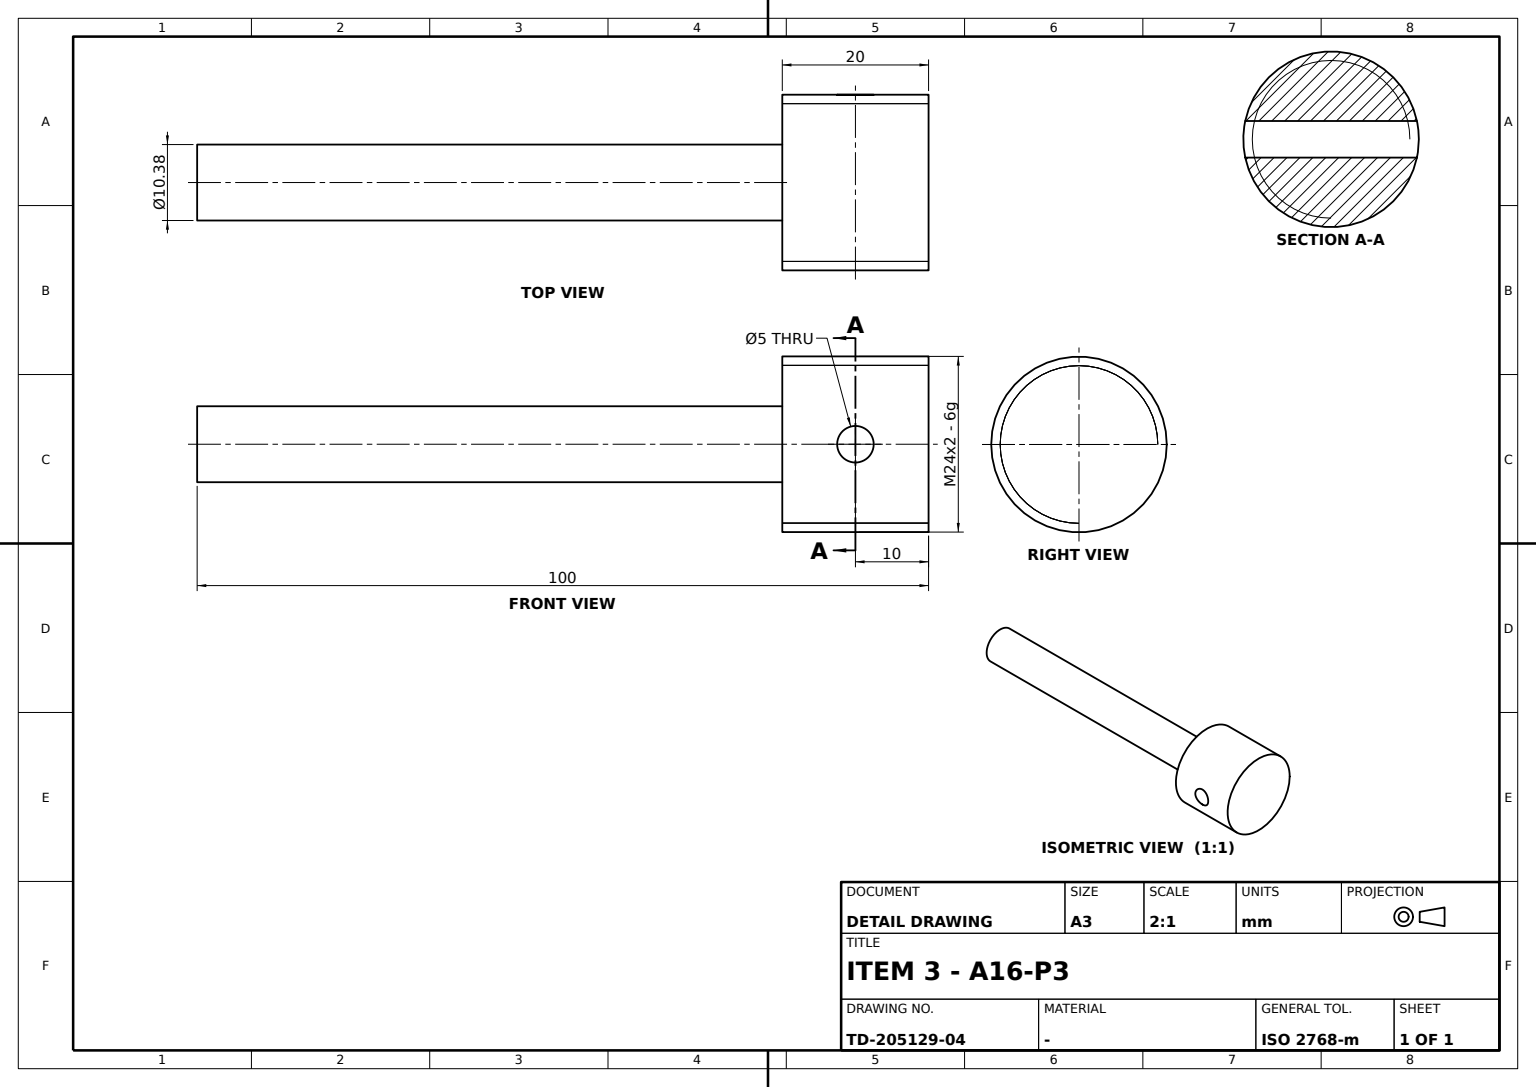
ISO-10303-21;
HEADER;
FILE_DESCRIPTION((''),'2;1');
FILE_NAME('','',(''),(''),'','','');
FILE_SCHEMA(('AUTOMOTIVE_DESIGN'));
ENDSEC;
DATA;
#1=APPLICATION_CONTEXT('');
#2=PRODUCT_CONTEXT('',#1,'mechanical');
#3=PRODUCT('','','',(#2));
#4=PRODUCT_DEFINITION_FORMATION('','',#3);
#5=PRODUCT_DEFINITION_CONTEXT('',#1,'design');
#6=PRODUCT_DEFINITION('','',#4,#5);
#7=PRODUCT_DEFINITION_SHAPE('','',#6);
#8=(LENGTH_UNIT()NAMED_UNIT(*)SI_UNIT(.MILLI.,.METRE.));
#9=(NAMED_UNIT(*)PLANE_ANGLE_UNIT()SI_UNIT($,.RADIAN.));
#10=(NAMED_UNIT(*)SI_UNIT($,.STERADIAN.)SOLID_ANGLE_UNIT());
#11=UNCERTAINTY_MEASURE_WITH_UNIT(LENGTH_MEASURE(0.005),#8,'distance_accuracy_value','');
#12=(GEOMETRIC_REPRESENTATION_CONTEXT(3)GLOBAL_UNCERTAINTY_ASSIGNED_CONTEXT((#11))GLOBAL_UNIT_ASSIGNED_CONTEXT((#8,#9,#10))REPRESENTATION_CONTEXT('',''));
#13=CARTESIAN_POINT('',(0.,12.,100.));
#14=VERTEX_POINT('',#13);
#15=CARTESIAN_POINT('',(0.,0.,100.));
#16=DIRECTION('',(0.,0.,-1.));
#17=DIRECTION('',(0.,1.,0.));
#18=AXIS2_PLACEMENT_3D('',#15,#16,#17);
#19=CIRCLE('',#18,12.);
#20=EDGE_CURVE('',#14,#14,#19,.T.);
#21=ORIENTED_EDGE('',*,*,#20,.F.);
#22=EDGE_LOOP('',(#21));
#23=FACE_BOUND('',#22,.T.);
#24=DIRECTION('',(1.,0.,0.));
#25=AXIS2_PLACEMENT_3D('',#13,#16,#24);
#26=PLANE('',#25);
#27=ADVANCED_FACE('',(#23),#26,.F.);
#28=CARTESIAN_POINT('',(0.,5.188,0.));
#29=VERTEX_POINT('',#28);
#30=CARTESIAN_POINT('',(0.,0.,0.));
#31=AXIS2_PLACEMENT_3D('',#30,#16,#17);
#32=CIRCLE('',#31,5.188);
#33=EDGE_CURVE('',#29,#29,#32,.T.);
#34=ORIENTED_EDGE('',*,*,#33,.F.);
#35=EDGE_LOOP('',(#34));
#36=FACE_BOUND('',#35,.T.);
#37=CARTESIAN_POINT('',(0.,5.188,80.));
#38=VERTEX_POINT('',#37);
#39=CARTESIAN_POINT('',(0.,0.,80.));
#40=AXIS2_PLACEMENT_3D('',#39,#16,#17);
#41=CIRCLE('',#40,5.188);
#42=EDGE_CURVE('',#38,#38,#41,.T.);
#43=ORIENTED_EDGE('',*,*,#42,.T.);
#44=EDGE_LOOP('',(#43));
#45=FACE_BOUND('',#44,.T.);
#46=CARTESIAN_POINT('',(0.,0.,50.));
#47=AXIS2_PLACEMENT_3D('',#46,#16,#24);
#48=CYLINDRICAL_SURFACE('',#47,5.188);
#49=ADVANCED_FACE('',(#36,#45),#48,.T.);
#50=ORIENTED_EDGE('',*,*,#33,.T.);
#51=EDGE_LOOP('',(#50));
#52=FACE_BOUND('',#51,.T.);
#53=AXIS2_PLACEMENT_3D('',#30,#16,#24);
#54=PLANE('',#53);
#55=ADVANCED_FACE('',(#52),#54,.T.);
#56=ORIENTED_EDGE('',*,*,#42,.F.);
#57=EDGE_LOOP('',(#56));
#58=FACE_BOUND('',#57,.T.);
#59=CARTESIAN_POINT('',(0.,12.,80.));
#60=VERTEX_POINT('',#59);
#61=CIRCLE('',#40,12.);
#62=EDGE_CURVE('',#60,#60,#61,.T.);
#63=ORIENTED_EDGE('',*,*,#62,.T.);
#64=EDGE_LOOP('',(#63));
#65=FACE_BOUND('',#64,.T.);
#66=AXIS2_PLACEMENT_3D('',#37,#16,#24);
#67=PLANE('',#66);
#68=ADVANCED_FACE('',(#58,#65),#67,.T.);
#69=CARTESIAN_POINT('',(2.5,-11.736695,90.));
#70=VERTEX_POINT('',#69);
#71=CARTESIAN_POINT('',(1.958372,-11.870043,91.960573));
#72=CARTESIAN_POINT('',(2.770873,-11.670071,89.999616));
#73=CARTESIAN_POINT('',(1.958134,-11.869843,88.040963));
#74=CARTESIAN_POINT('',(0.003168,-12.065028,87.229905));
#75=CARTESIAN_POINT('',(-1.958354,-11.870046,88.03942));
#76=CARTESIAN_POINT('',(-2.770873,-11.670071,90.000335));
#77=CARTESIAN_POINT('',(-1.958152,-11.869839,91.95903));
#78=CARTESIAN_POINT('',(-0.003168,-12.065029,92.770098));
#79=B_SPLINE_CURVE_WITH_KNOTS('',3,(#71,#72,#73,#74,#75,#76,#77,#78,#71,#72,#73),.UNSPECIFIED.,.T.,.F.,(1,1,1,1,1,1,1,1,1,1,1,1,1,1,1),(-0.005876569,-0.003917713,-0.001958856,0.,0.001958856,0.003917713,0.005876569,0.007835425,0.009794281,0.011753138,0.013711994,0.01567085,0.017629707,0.019588563,0.021547419),.UNSPECIFIED.);
#80=EDGE_CURVE('',#70,#70,#79,.T.);
#81=ORIENTED_EDGE('',*,*,#80,.F.);
#82=EDGE_LOOP('',(#81));
#83=FACE_BOUND('',#82,.T.);
#84=CARTESIAN_POINT('',(-2.5,11.736695,90.));
#85=VERTEX_POINT('',#84);
#86=CARTESIAN_POINT('',(-1.958372,11.870043,88.039427));
#87=CARTESIAN_POINT('',(-2.770873,11.670071,90.000384));
#88=CARTESIAN_POINT('',(-1.958134,11.869843,91.959037));
#89=CARTESIAN_POINT('',(-0.003168,12.065028,92.770095));
#90=CARTESIAN_POINT('',(1.958354,11.870046,91.96058));
#91=CARTESIAN_POINT('',(2.770873,11.670071,89.999665));
#92=CARTESIAN_POINT('',(1.958152,11.869839,88.04097));
#93=CARTESIAN_POINT('',(0.003168,12.065029,87.229902));
#94=B_SPLINE_CURVE_WITH_KNOTS('',3,(#86,#87,#88,#89,#90,#91,#92,#93,#86,#87,#88),.UNSPECIFIED.,.T.,.F.,(1,1,1,1,1,1,1,1,1,1,1,1,1,1,1),(-0.005876569,-0.003917713,-0.001958856,0.,0.001958856,0.003917713,0.005876569,0.007835425,0.009794281,0.011753138,0.013711994,0.01567085,0.017629707,0.019588563,0.021547419),.UNSPECIFIED.);
#95=EDGE_CURVE('',#85,#85,#94,.F.);
#96=ORIENTED_EDGE('',*,*,#95,.F.);
#97=EDGE_LOOP('',(#96));
#98=FACE_BOUND('',#97,.T.);
#99=CARTESIAN_POINT('',(0.,0.,90.));
#100=DIRECTION('',(-1.,0.,0.));
#101=AXIS2_PLACEMENT_3D('',#99,#17,#100);
#102=CYLINDRICAL_SURFACE('',#101,2.5);
#103=ADVANCED_FACE('',(#83,#98),#102,.F.);
#104=ORIENTED_EDGE('',*,*,#80,.T.);
#105=EDGE_LOOP('',(#104));
#106=FACE_BOUND('',#105,.T.);
#107=ORIENTED_EDGE('',*,*,#95,.T.);
#108=EDGE_LOOP('',(#107));
#109=FACE_BOUND('',#108,.T.);
#110=ORIENTED_EDGE('',*,*,#20,.T.);
#111=EDGE_LOOP('',(#110));
#112=FACE_BOUND('',#111,.T.);
#113=ORIENTED_EDGE('',*,*,#62,.F.);
#114=EDGE_LOOP('',(#113));
#115=FACE_BOUND('',#114,.T.);
#116=CYLINDRICAL_SURFACE('',#47,12.);
#117=ADVANCED_FACE('',(#106,#109,#112,#115),#116,.T.);
#118=CLOSED_SHELL('',(#27,#49,#55,#68,#103,#117));
#119=MANIFOLD_SOLID_BREP('',#118);
#120=ADVANCED_BREP_SHAPE_REPRESENTATION('',(#119),#12);
#121=SHAPE_DEFINITION_REPRESENTATION(#7,#120);
ENDSEC;
END-ISO-10303-21;
